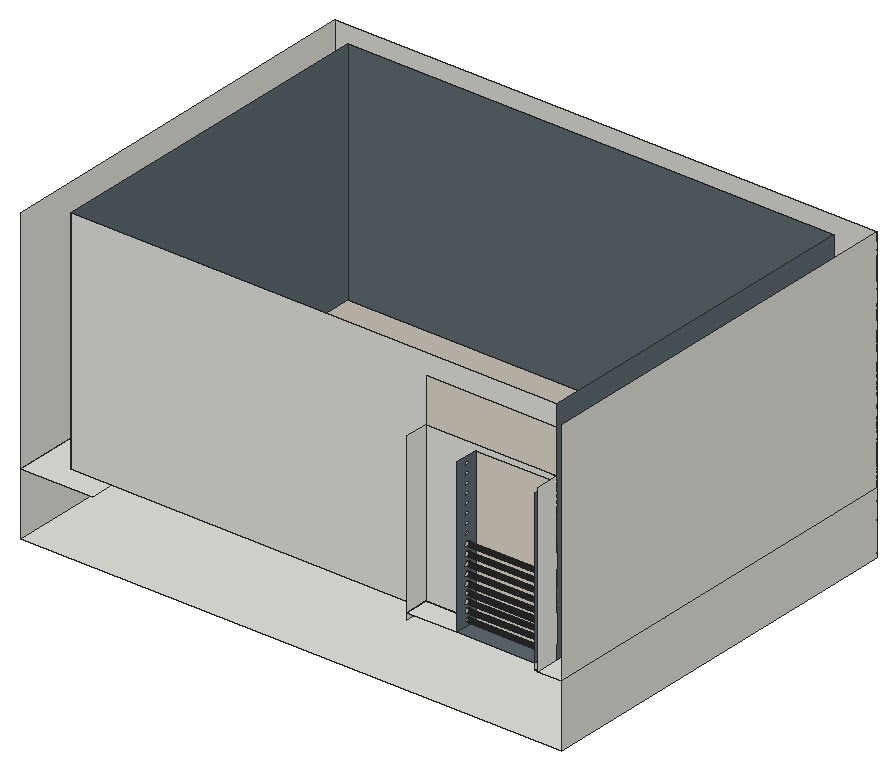
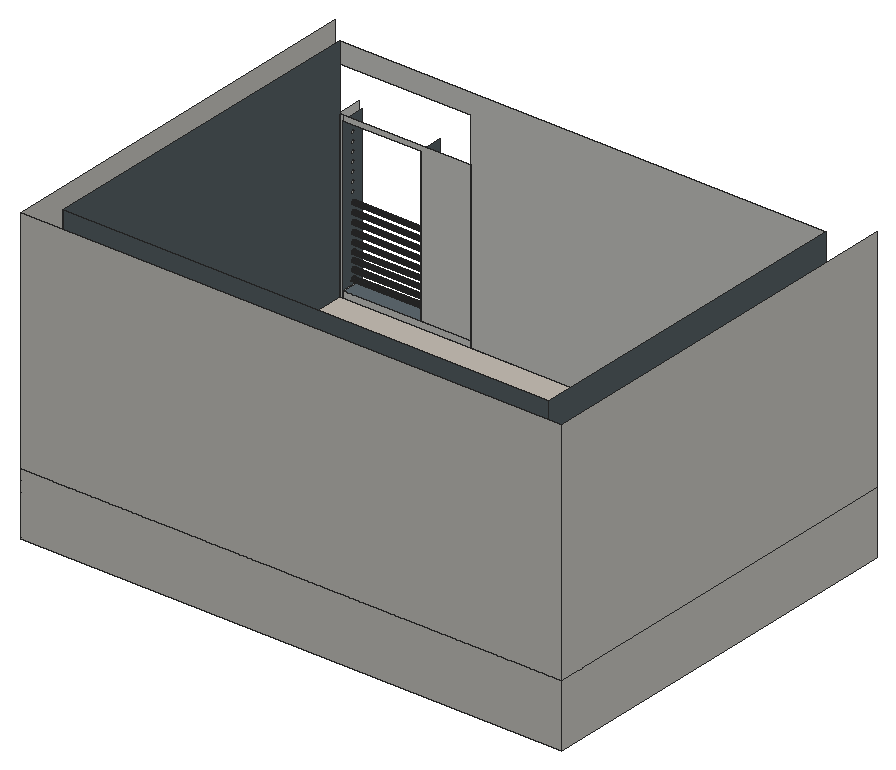
# SketchUp Ruby script. Lengths in inches.
U = 1.inch
M = Sketchup.active_model
def pt(a) = Geom::Point3d.new(a.map { |v| v * U })
def face(e, loops, mat)
  f = e.add_face(loops[0].map { |a| pt(a) })
  loops[1..].each { |l| e.add_face(l.map { |a| pt(a) }).erase! }
  f.material = f.back_material = mat if mat
  f
end
# faces: each face lists its corners as indices into pts; further lists are holes
def faces(e, pts, list, mat = nil) = list.each { |f| face(e, (f[0].is_a?(Array) ? f : [f]).map { |l| l.map { |i| pts[i] } }, mat) }
# xy, xz, yz: faces in a plane at the given z, y or x. An outline is a flat list of corners, or four numbers for a rectangle; further outlines are holes
def ring(l) = l.size == 4 ? [[l[0], l[1]], [l[2], l[1]], [l[2], l[3]], [l[0], l[3]]] : l.each_slice(2).to_a
def flat(e, list, mat, &to3) = list.each { |f| face(e, (f[0].is_a?(Array) ? f : [f]).map { |l| ring(l).map { |u, v| to3.(u, v) } }, mat) }
def xy(e, z, list, mat = nil) = flat(e, list, mat) { |x, y| [x, y, z] }
def xz(e, y, list, mat = nil) = flat(e, list, mat) { |x, z| [x, y, z] }
def yz(e, x, list, mat = nil) = flat(e, list, mat) { |y, z| [x, y, z] }
def lines(e, pts, list) = list.each { |a, b| e.add_line(pt(pts[a]), pt(pts[b])) }
# prism: a flat outline (further loops are holes) pulled along v
def prism(e, loops, v, mat = nil)
  f = face(e, loops, mat); d = Geom::Vector3d.new(v.map { |x| x * U })
  f.pushpull(f.normal.samedirection?(d) ? d.length : -d.length)
end
def box(e, o, s, mat = nil) = prism(e, [[o, [o[0] + s[0], o[1], o[2]], [o[0] + s[0], o[1] + s[1], o[2]], [o[0], o[1] + s[1], o[2]]]], [0, 0, s[2]], mat)
def at(x, y, z, deg = 0) = Geom::Transformation.translation(pt([x, y, z])) * Geom::Transformation.rotation(ORIGIN, Z_AXIS, deg.degrees)
def axes(o, x, y, z) = Geom::Transformation.new([*x, 0, *y, 0, *z, 0, *pt(o).to_a, 1])
def part(name) = M.definitions.add(name)
# library, detail: a bought-in or finely detailed component or shape, given as its bounding box
def library(name, o, s) = part(name).tap { |d| box(d.entities, o, s) }
def detail(e, o, s) = box(e.add_group.entities, o, s)
def put(e, d, t, mat = nil) = e.add_instance(d, t).tap { |i| i.material = mat if mat }
def group(e, t, mat = nil) = e.add_group.tap { |g| g.transformation = t; g.material = mat if mat }.entities
root = M.entities
M.materials.add("[Field Rectangle Tile]").color = [196, 189, 179]
M.materials.add("[Formica Laminate Dark]").color = [50, 53, 60]
M.materials.add("[Formica Speckled Grey]").color = [94, 105, 111]
M.materials.add("[Terrazzo Tile Light]").color = [219, 217, 210]
xy(root,0,[[57.16,175.06,340.49,380.73]])
xy(root,32.8125,[[57.16,175.06,57.16,380.73,340.49,380.73,340.49,175.06,328.05,175.06,328.05,368.29,73.72,368.29,73.72,187.5,94.84,187.5,94.84,175.06],[326.14,175.06,328.05,187.5]])
xy(root,32.8125,[[73.72,187.5,328.05,368.29]],"[Field Rectangle Tile]")
xy(root,36.375,[[259.37,175.06,285.76,187.5]])
xy(root,36.375,[[285.76,175.06,326.14,187.5]],"[Formica Speckled Grey]")
xz(root,187.5,[[73.72,32.8125,73.72,152.8125,328.05,152.8125,328.05,142.25,259.37,142.25,259.37,32.8125],[259.37,32.8125,326.14,36.375],[326.14,32.8125,328.05,119],[259.37,36.375,259.37,119,326.14,119,326.14,116.03,285.76,116.03,285.76,36.375]])
xz(root,368.29,[[73.72,32.8125,328.05,152.8125]],"[Formica Speckled Grey]")
xz(root,380.73,[[57.16,0,340.49,32.8125],[57.16,32.8125,340.49,152.8125]],"[Terrazzo Tile Light]")
yz(root,57.16,[[175.06,0,380.73,32.8125],[175.06,32.8125,380.73,152.8125]],"[Terrazzo Tile Light]")
yz(root,73.72,[[187.5,32.8125,368.29,152.8125]],"[Formica Speckled Grey]")
yz(root,259.37,[[175.06,32.8125,187.5,36.375],[175.06,36.375,187.5,119]])
yz(root,285.76,[[181.41,38.33,181.12,38.37,180.85,38.48,180.62,38.66,180.4375,38.9,180.33,39.17,180.29,39.46,180.33,39.75,180.4375,40.02,180.62,40.25,180.85,40.43,181.12,40.55,181.41,40.58,181.7,40.55,181.98,40.43,182.21,40.25,182.39,40.02,182.5,39.75,182.54,39.46,182.5,39.17,182.39,38.9,182.21,38.66,181.98,38.48,181.7,38.37],[181.28,42.8,180.99,42.84,180.72,42.95,180.49,43.125,180.31,43.36,180.2,43.63,180.16,43.92,180.2,44.21,180.31,44.48,180.49,44.72,180.72,44.9,180.99,45.01,181.28,45.05,181.57,45.01,181.84,44.9,182.08,44.72,182.26,44.48,182.37,44.21,182.41,43.92,182.37,43.63,182.26,43.36,182.08,43.125,181.84,42.95,181.57,42.84],[181.25,47.03,180.96,47.07,180.6875,47.18,180.45,47.36,180.28,47.59,180.16,47.86,180.125,48.15,180.16,48.44,180.28,48.72,180.45,48.95,180.6875,49.13,180.96,49.24,181.25,49.28,181.54,49.24,181.8125,49.13,182.05,48.95,182.22,48.72,182.34,48.44,182.375,48.15,182.34,47.86,182.22,47.59,182.05,47.36,181.8125,47.18,181.54,47.07],[181.25,51.09,180.96,51.13,180.6875,51.24,180.45,51.42,180.28,51.65,180.16,51.92,180.125,52.22,180.16,52.51,180.28,52.78,180.45,53.01,180.6875,53.19,180.96,53.3,181.25,53.34,181.54,53.3,181.8125,53.19,182.05,53.01,182.22,52.78,182.34,52.51,182.375,52.22,182.34,51.92,182.22,51.65,182.05,51.42,181.8125,51.24,181.54,51.13],[181.25,55.47,180.96,55.5,180.6875,55.62,180.45,55.8,180.28,56.03,180.16,56.3,180.125,56.59,180.16,56.88,180.28,57.15,180.45,57.39,180.6875,57.57,180.96,57.68,181.25,57.72,181.54,57.68,181.8125,57.57,182.05,57.39,182.22,57.15,182.34,56.88,182.375,56.59,182.34,56.3,182.22,56.03,182.05,55.8,181.8125,55.62,181.54,55.5],
  [181.25,60.15,180.96,60.19,180.6875,60.3,180.45,60.48,180.28,60.72,180.16,60.99,180.125,61.28,180.16,61.57,180.28,61.84,180.45,62.07,180.6875,62.25,180.96,62.37,181.25,62.4,181.54,62.37,181.8125,62.25,182.05,62.07,182.22,61.84,182.34,61.57,182.375,61.28,182.34,60.99,182.22,60.72,182.05,60.48,181.8125,60.3,181.54,60.19],[181.25,64.84,180.96,64.88,180.6875,64.99,180.45,65.17,180.28,65.4,180.16,65.67,180.125,65.97,180.16,66.26,180.28,66.53,180.45,66.76,180.6875,66.94,180.96,67.05,181.25,67.09,181.54,67.05,181.8125,66.94,182.05,66.76,182.22,66.53,182.34,66.26,182.375,65.97,182.34,65.67,182.22,65.4,182.05,65.17,181.8125,64.99,181.54,64.88],[181.25,69.53,180.96,69.57,180.6875,69.68,180.45,69.86,180.28,70.09,180.16,70.36,180.125,70.65,180.16,70.94,180.28,71.22,180.45,71.45,180.6875,71.63,180.96,71.74,181.25,71.78,181.54,71.74,181.8125,71.63,182.05,71.45,182.22,71.22,182.34,70.94,182.375,70.65,182.34,70.36,182.22,70.09,182.05,69.86,181.8125,69.68,181.54,69.57],[181.25,74.22,180.96,74.25,180.6875,74.37,180.45,74.55,180.28,74.78,180.16,75.05,180.125,75.34,180.16,75.63,180.28,75.9,180.45,76.14,180.6875,76.32,180.96,76.43,181.25,76.47,181.54,76.43,181.8125,76.32,182.05,76.14,182.22,75.9,182.34,75.63,182.375,75.34,182.34,75.05,182.22,74.78,182.05,74.55,181.8125,74.37,181.54,74.25]])
yz(root,285.76,[[[175.06,36.375,187.5,116.03],[181.25,107.03,180.96,107.07,180.6875,107.18,180.45,107.36,180.28,107.59,180.16,107.86,180.125,108.15,180.16,108.44,180.28,108.72,180.45,108.95,180.6875,109.13,180.96,109.24,181.25,109.28,181.54,109.24,181.8125,109.13,182.05,108.95,182.22,108.72,182.34,108.44,182.375,108.15,182.34,107.86,182.22,107.59,182.05,107.36,181.8125,107.18,181.54,107.07],[181.25,102.34,180.96,102.38,180.6875,102.49,180.45,102.67,180.28,102.9,180.16,103.17,180.125,103.47,180.16,103.76,180.28,104.03,180.45,104.26,180.6875,104.44,180.96,104.55,181.25,104.59,181.54,104.55,181.8125,104.44,182.05,104.26,182.22,104.03,182.34,103.76,182.375,103.47,182.34,103.17,182.22,102.9,182.05,102.67,181.8125,102.49,181.54,102.38],[181.25,97.65,180.96,97.69,180.6875,97.8,180.45,97.98,180.28,98.22,180.16,98.49,180.125,98.78,180.16,99.07,180.28,99.34,180.45,99.57,180.6875,99.75,180.96,99.87,181.25,99.9,181.54,99.87,181.8125,99.75,182.05,99.57,182.22,99.34,182.34,99.07,182.375,98.78,182.34,98.49,182.22,98.22,182.05,97.98,181.8125,97.8,181.54,97.69],[181.25,92.97,180.96,93,180.6875,93.12,180.45,93.3,180.28,93.53,180.16,93.8,180.125,94.09,180.16,94.38,180.28,94.65,180.45,94.89,180.6875,95.07,180.96,95.18,181.25,95.22,181.54,95.18,181.8125,95.07,182.05,94.89,182.22,94.65,182.34,94.38,182.375,94.09,182.34,93.8,182.22,93.53,182.05,93.3,181.8125,93.12,181.54,93],[181.25,88.28,180.96,88.32,180.6875,88.43,180.45,88.61,180.28,88.84,180.16,89.11,180.125,89.4,180.16,89.69,180.28,89.97,180.45,90.2,180.6875,90.38,180.96,90.49,181.25,90.53,181.54,90.49,181.8125,90.38,182.05,90.2,182.22,89.97,182.34,89.69,182.375,89.4,182.34,89.11,182.22,88.84,182.05,88.61,181.8125,88.43,181.54,88.32],[181.25,83.59,180.96,83.63,180.6875,83.74,180.45,83.92,180.28,84.15,180.16,84.42,180.125,84.72,180.16,85.01,180.28,85.28,180.45,85.51,180.6875,85.69,180.96,85.8,181.25,85.84,181.54,85.8,181.8125,85.69,182.05,85.51,182.22,85.28,182.34,85.01,182.375,84.72,182.34,84.42,182.22,84.15,182.05,83.92,181.8125,83.74,181.54,83.63],[181.25,78.9,180.96,78.94,180.6875,79.05,180.45,79.23,180.28,79.47,180.16,79.74,180.125,80.03,180.16,80.32,180.28,80.59,180.45,80.82,180.6875,81,180.96,81.12,181.25,81.15,181.54,81.12,181.8125,81,182.05,80.82,182.22,80.59,182.34,80.32,182.375,80.03,182.34,79.74,182.22,79.47,182.05,79.23,181.8125,79.05,181.54,78.94],[181.25,74.22,180.96,74.25,180.6875,74.37,180.45,74.55,180.28,74.78,180.16,75.05,180.125,75.34,180.16,75.63,180.28,75.9,180.45,76.14,180.6875,76.32,180.96,76.43,181.25,76.47,181.54,76.43,181.8125,76.32,182.05,76.14,182.22,75.9,182.34,75.63,182.375,75.34,182.34,75.05,182.22,74.78,182.05,74.55,181.8125,74.37,181.54,74.25],[181.25,69.53,180.96,69.57,180.6875,69.68,180.45,69.86,180.28,70.09,180.16,70.36,180.125,70.65,180.16,70.94,180.28,71.22,180.45,71.45,180.6875,71.63,180.96,71.74,181.25,71.78,181.54,71.74,181.8125,71.63,182.05,71.45,182.22,71.22,182.34,70.94,182.375,70.65,182.34,70.36,182.22,70.09,182.05,69.86,181.8125,69.68,181.54,69.57],[181.25,64.84,180.96,64.88,180.6875,64.99,180.45,65.17,180.28,65.4,180.16,65.67,180.125,65.97,180.16,66.26,180.28,66.53,180.45,66.76,180.6875,66.94,180.96,67.05,181.25,67.09,181.54,67.05,181.8125,66.94,182.05,66.76,182.22,66.53,182.34,66.26,182.375,65.97,182.34,65.67,182.22,65.4,182.05,65.17,181.8125,64.99,181.54,64.88],[181.25,60.15,180.96,60.19,180.6875,60.3,180.45,60.48,180.28,60.72,180.16,60.99,180.125,61.28,180.16,61.57,180.28,61.84,180.45,62.07,180.6875,62.25,180.96,62.37,181.25,62.4,181.54,62.37,181.8125,62.25,182.05,62.07,182.22,61.84,182.34,61.57,182.375,61.28,182.34,60.99,182.22,60.72,182.05,60.48,181.8125,60.3,181.54,60.19],[181.25,55.47,180.96,55.5,180.6875,55.62,180.45,55.8,180.28,56.03,180.16,56.3,180.125,56.59,180.16,56.88,180.28,57.15,180.45,57.39,180.6875,57.57,180.96,57.68,181.25,57.72,181.54,57.68,181.8125,57.57,182.05,57.39,182.22,57.15,182.34,56.88,182.375,56.59,182.34,56.3,182.22,56.03,182.05,55.8,181.8125,55.62,181.54,55.5],[181.41,38.33,181.12,38.37,180.85,38.48,180.62,38.66,180.4375,38.9,180.33,39.17,180.29,39.46,180.33,39.75,180.4375,40.02,180.62,40.25,180.85,40.43,181.12,40.55,181.41,40.58,181.7,40.55,181.98,40.43,182.21,40.25,182.39,40.02,182.5,39.75,182.54,39.46,182.5,39.17,182.39,38.9,182.21,38.66,181.98,38.48,181.7,38.37],[181.25,51.09,180.96,51.13,180.6875,51.24,180.45,51.42,180.28,51.65,180.16,51.92,180.125,52.22,180.16,52.51,180.28,52.78,180.45,53.01,180.6875,53.19,180.96,53.3,181.25,53.34,181.54,53.3,181.8125,53.19,182.05,53.01,182.22,52.78,182.34,52.51,182.375,52.22,182.34,51.92,182.22,51.65,182.05,51.42,181.8125,51.24,181.54,51.13],[181.28,42.8,180.99,42.84,180.72,42.95,180.49,43.125,180.31,43.36,180.2,43.63,180.16,43.92,180.2,44.21,180.31,44.48,180.49,44.72,180.72,44.9,180.99,45.01,181.28,45.05,181.57,45.01,181.84,44.9,182.08,44.72,182.26,44.48,182.37,44.21,182.41,43.92,182.37,43.63,182.26,43.36,182.08,43.125,181.84,42.95,181.57,42.84],[181.25,47.03,180.96,47.07,180.6875,47.18,180.45,47.36,180.28,47.59,180.16,47.86,180.125,48.15,180.16,48.44,180.28,48.72,180.45,48.95,180.6875,49.13,180.96,49.24,181.25,49.28,181.54,49.24,181.8125,49.13,182.05,48.95,182.22,48.72,182.34,48.44,182.375,48.15,182.34,47.86,182.22,47.59,182.05,47.36,181.8125,47.18,181.54,47.07],[181.25,111.72,180.96,111.75,180.6875,111.87,180.45,112.05,180.28,112.28,180.16,112.55,180.125,112.84,180.16,113.13,180.28,113.4,180.45,113.64,180.6875,113.82,180.96,113.93,181.25,113.97,181.54,113.93,181.8125,113.82,182.05,113.64,182.22,113.4,182.34,113.13,182.375,112.84,182.34,112.55,182.22,112.28,182.05,112.05,181.8125,111.87,181.54,111.75]]],"[Formica Speckled Grey]")
yz(root,326.14,[[175.06,32.8125,187.5,36.375]])
yz(root,326.14,[[[175.06,36.375,187.5,116.03],[181.25,111.72,181.54,111.75,181.8125,111.87,182.05,112.05,182.22,112.28,182.34,112.55,182.375,112.84,182.34,113.13,182.22,113.4,182.05,113.64,181.8125,113.82,181.54,113.93,181.25,113.97,180.96,113.93,180.6875,113.82,180.45,113.64,180.28,113.4,180.16,113.13,180.125,112.84,180.16,112.55,180.28,112.28,180.45,112.05,180.6875,111.87,180.96,111.75],[181.25,107.03,181.54,107.07,181.8125,107.18,182.05,107.36,182.22,107.59,182.34,107.86,182.375,108.15,182.34,108.44,182.22,108.72,182.05,108.95,181.8125,109.13,181.54,109.24,181.25,109.28,180.96,109.24,180.6875,109.13,180.45,108.95,180.28,108.72,180.16,108.44,180.125,108.15,180.16,107.86,180.28,107.59,180.45,107.36,180.6875,107.18,180.96,107.07],[181.25,102.34,181.54,102.38,181.8125,102.49,182.05,102.67,182.22,102.9,182.34,103.17,182.375,103.47,182.34,103.76,182.22,104.03,182.05,104.26,181.8125,104.44,181.54,104.55,181.25,104.59,180.96,104.55,180.6875,104.44,180.45,104.26,180.28,104.03,180.16,103.76,180.125,103.47,180.16,103.17,180.28,102.9,180.45,102.67,180.6875,102.49,180.96,102.38],[181.25,97.65,181.54,97.69,181.8125,97.8,182.05,97.98,182.22,98.22,182.34,98.49,182.375,98.78,182.34,99.07,182.22,99.34,182.05,99.57,181.8125,99.75,181.54,99.87,181.25,99.9,180.96,99.87,180.6875,99.75,180.45,99.57,180.28,99.34,180.16,99.07,180.125,98.78,180.16,98.49,180.28,98.22,180.45,97.98,180.6875,97.8,180.96,97.69],[181.25,92.97,181.54,93,181.8125,93.12,182.05,93.3,182.22,93.53,182.34,93.8,182.375,94.09,182.34,94.38,182.22,94.65,182.05,94.89,181.8125,95.07,181.54,95.18,181.25,95.22,180.96,95.18,180.6875,95.07,180.45,94.89,180.28,94.65,180.16,94.38,180.125,94.09,180.16,93.8,180.28,93.53,180.45,93.3,180.6875,93.12,180.96,93],[181.25,88.28,181.54,88.32,181.8125,88.43,182.05,88.61,182.22,88.84,182.34,89.11,182.375,89.4,182.34,89.69,182.22,89.97,182.05,90.2,181.8125,90.38,181.54,90.49,181.25,90.53,180.96,90.49,180.6875,90.38,180.45,90.2,180.28,89.97,180.16,89.69,180.125,89.4,180.16,89.11,180.28,88.84,180.45,88.61,180.6875,88.43,180.96,88.32],[181.25,83.59,181.54,83.63,181.8125,83.74,182.05,83.92,182.22,84.15,182.34,84.42,182.375,84.72,182.34,85.01,182.22,85.28,182.05,85.51,181.8125,85.69,181.54,85.8,181.25,85.84,180.96,85.8,180.6875,85.69,180.45,85.51,180.28,85.28,180.16,85.01,180.125,84.72,180.16,84.42,180.28,84.15,180.45,83.92,180.6875,83.74,180.96,83.63],[181.25,78.9,181.54,78.94,181.8125,79.05,182.05,79.23,182.22,79.47,182.34,79.74,182.375,80.03,182.34,80.32,182.22,80.59,182.05,80.82,181.8125,81,181.54,81.12,181.25,81.15,180.96,81.12,180.6875,81,180.45,80.82,180.28,80.59,180.16,80.32,180.125,80.03,180.16,79.74,180.28,79.47,180.45,79.23,180.6875,79.05,180.96,78.94],[181.25,74.22,181.54,74.25,181.8125,74.37,182.05,74.55,182.22,74.78,182.34,75.05,182.375,75.34,182.34,75.63,182.22,75.9,182.05,76.14,181.8125,76.32,181.54,76.43,181.25,76.47,180.96,76.43,180.6875,76.32,180.45,76.14,180.28,75.9,180.16,75.63,180.125,75.34,180.16,75.05,180.28,74.78,180.45,74.55,180.6875,74.37,180.96,74.25],[181.25,69.53,181.54,69.57,181.8125,69.68,182.05,69.86,182.22,70.09,182.34,70.36,182.375,70.65,182.34,70.94,182.22,71.22,182.05,71.45,181.8125,71.63,181.54,71.74,181.25,71.78,180.96,71.74,180.6875,71.63,180.45,71.45,180.28,71.22,180.16,70.94,180.125,70.65,180.16,70.36,180.28,70.09,180.45,69.86,180.6875,69.68,180.96,69.57],[181.25,64.84,181.54,64.88,181.8125,64.99,182.05,65.17,182.22,65.4,182.34,65.67,182.375,65.97,182.34,66.26,182.22,66.53,182.05,66.76,181.8125,66.94,181.54,67.05,181.25,67.09,180.96,67.05,180.6875,66.94,180.45,66.76,180.28,66.53,180.16,66.26,180.125,65.97,180.16,65.67,180.28,65.4,180.45,65.17,180.6875,64.99,180.96,64.88],[181.25,60.15,181.54,60.19,181.8125,60.3,182.05,60.48,182.22,60.72,182.34,60.99,182.375,61.28,182.34,61.57,182.22,61.84,182.05,62.07,181.8125,62.25,181.54,62.37,181.25,62.4,180.96,62.37,180.6875,62.25,180.45,62.07,180.28,61.84,180.16,61.57,180.125,61.28,180.16,60.99,180.28,60.72,180.45,60.48,180.6875,60.3,180.96,60.19],[181.25,55.47,181.54,55.5,181.8125,55.62,182.05,55.8,182.22,56.03,182.34,56.3,182.375,56.59,182.34,56.88,182.22,57.15,182.05,57.39,181.8125,57.57,181.54,57.68,181.25,57.72,180.96,57.68,180.6875,57.57,180.45,57.39,180.28,57.15,180.16,56.88,180.125,56.59,180.16,56.3,180.28,56.03,180.45,55.8,180.6875,55.62,180.96,55.5],[181.25,51.09,181.54,51.13,181.8125,51.24,182.05,51.42,182.22,51.65,182.34,51.92,182.375,52.22,182.34,52.51,182.22,52.78,182.05,53.01,181.8125,53.19,181.54,53.3,181.25,53.34,180.96,53.3,180.6875,53.19,180.45,53.01,180.28,52.78,180.16,52.51,180.125,52.22,180.16,51.92,180.28,51.65,180.45,51.42,180.6875,51.24,180.96,51.13],[181.25,47.03,181.54,47.07,181.8125,47.18,182.05,47.36,182.22,47.59,182.34,47.86,182.375,48.15,182.34,48.44,182.22,48.72,182.05,48.95,181.8125,49.13,181.54,49.24,181.25,49.28,180.96,49.24,180.6875,49.13,180.45,48.95,180.28,48.72,180.16,48.44,180.125,48.15,180.16,47.86,180.28,47.59,180.45,47.36,180.6875,47.18,180.96,47.07],[181.28,42.8,181.57,42.84,181.84,42.95,182.08,43.125,182.26,43.36,182.37,43.63,182.41,43.92,182.37,44.21,182.26,44.48,182.08,44.72,181.84,44.9,181.57,45.01,181.28,45.05,180.99,45.01,180.72,44.9,180.49,44.72,180.31,44.48,180.2,44.21,180.16,43.92,180.2,43.63,180.31,43.36,180.49,43.125,180.72,42.95,180.99,42.84],[181.41,38.33,181.7,38.37,181.98,38.48,182.21,38.66,182.39,38.9,182.5,39.17,182.54,39.46,182.5,39.75,182.39,40.02,182.21,40.25,181.98,40.43,181.7,40.55,181.41,40.58,181.12,40.55,180.85,40.43,180.62,40.25,180.4375,40.02,180.33,39.75,180.29,39.46,180.33,39.17,180.4375,38.9,180.62,38.66,180.85,38.48,181.12,38.37]]],"[Formica Speckled Grey]")
yz(root,328.05,[[175.06,32.8125,187.5,119]])
yz(root,328.05,[[187.5,32.8125,368.29,152.8125]],"[Formica Speckled Grey]")
yz(root,340.49,[[175.06,0,380.73,32.8125],[175.06,32.8125,380.73,152.8125]],"[Terrazzo Tile Light]")
p = [[285.76,181.12,38.37],[285.76,181.41,38.33],[326.14,181.41,38.33],[326.14,181.12,38.37],[285.76,181.7,38.37],[326.14,181.7,38.37],
  [285.76,181.98,38.48],[326.14,181.98,38.48],[285.76,182.21,38.66],[326.14,182.21,38.66],[285.76,182.39,38.9],[326.14,182.39,38.9],
  [285.76,182.5,39.17],[326.14,182.5,39.17],[285.76,182.54,39.46],[326.14,182.54,39.46],[285.76,182.5,39.75],[326.14,182.5,39.75],
  [285.76,182.39,40.02],[326.14,182.39,40.02],[285.76,182.21,40.25],[326.14,182.21,40.25],[285.76,181.98,40.43],[326.14,181.98,40.43],
  [285.76,181.7,40.55],[326.14,181.7,40.55],[285.76,181.41,40.58],[285.76,181.12,40.55],[326.14,181.12,40.55],[326.14,181.41,40.58],
  [285.76,180.99,42.84],[285.76,181.28,42.8],[326.14,181.28,42.8],[326.14,180.99,42.84],[285.76,181.57,42.84],[326.14,181.57,42.84],
  [285.76,181.84,42.95],[326.14,181.84,42.95],[285.76,182.08,43.125],[326.14,182.08,43.125],[285.76,182.26,43.36],[326.14,182.26,43.36],
  [285.76,182.37,43.63],[326.14,182.37,43.63],[285.76,182.41,43.92],[326.14,182.41,43.92],[285.76,182.37,44.21],[326.14,182.37,44.21],
  [285.76,182.26,44.48],[326.14,182.26,44.48],[285.76,182.08,44.72],[326.14,182.08,44.72],[285.76,181.84,44.9],[326.14,181.84,44.9],
  [285.76,181.57,45.01],[326.14,181.57,45.01],[285.76,181.28,45.05],[285.76,180.99,45.01],[326.14,180.99,45.01],[326.14,181.28,45.05],
  [285.76,181.25,47.03],[285.76,181.54,47.07],[326.14,181.54,47.07],[326.14,181.25,47.03],[285.76,181.8125,47.18],[326.14,181.8125,47.18],
  [285.76,182.05,47.36],[326.14,182.05,47.36],[285.76,182.22,47.59],[326.14,182.22,47.59],[285.76,182.34,47.86],[326.14,182.34,47.86],
  [285.76,182.375,48.15],[326.14,182.375,48.15],[285.76,182.34,48.44],[326.14,182.34,48.44],[285.76,182.22,48.72],[326.14,182.22,48.72],
  [285.76,182.05,48.95],[326.14,182.05,48.95],[285.76,181.8125,49.13],[326.14,181.8125,49.13],[285.76,181.54,49.24],[326.14,181.54,49.24],
  [285.76,181.25,49.28],[326.14,181.25,49.28],[285.76,180.96,51.13],[285.76,181.25,51.09],[326.14,181.25,51.09],[326.14,180.96,51.13],
  [285.76,181.54,51.13],[326.14,181.54,51.13],[285.76,181.8125,51.24],[326.14,181.8125,51.24],[285.76,182.05,51.42],[326.14,182.05,51.42],
  [285.76,182.22,51.65],[326.14,182.22,51.65],[285.76,182.34,51.92],[326.14,182.34,51.92],[285.76,182.375,52.22],[326.14,182.375,52.22],
  [285.76,182.34,52.51],[326.14,182.34,52.51],[285.76,182.22,52.78],[326.14,182.22,52.78],[285.76,182.05,53.01],[326.14,182.05,53.01],
  [285.76,181.8125,53.19],[326.14,181.8125,53.19],[285.76,181.54,53.3],[326.14,181.54,53.3],[285.76,181.25,53.34],[285.76,180.96,53.3],
  [326.14,180.96,53.3],[326.14,181.25,53.34],[285.76,180.96,55.5],[285.76,181.25,55.47],[326.14,181.25,55.47],[326.14,180.96,55.5],
  [285.76,181.54,55.5],[326.14,181.54,55.5],[285.76,181.8125,55.62],[326.14,181.8125,55.62],[285.76,182.05,55.8],[326.14,182.05,55.8],
  [285.76,182.22,56.03],[326.14,182.22,56.03],[285.76,182.34,56.3],[326.14,182.34,56.3],[285.76,182.375,56.59],[326.14,182.375,56.59],
  [285.76,182.34,56.88],[326.14,182.34,56.88],[285.76,182.22,57.15],[326.14,182.22,57.15],[285.76,182.05,57.39],[326.14,182.05,57.39],
  [285.76,181.8125,57.57],[326.14,181.8125,57.57],[285.76,181.54,57.68],[326.14,181.54,57.68],[285.76,181.25,57.72],[285.76,180.96,57.68],
  [326.14,180.96,57.68],[326.14,181.25,57.72],[285.76,180.96,60.19],[285.76,181.25,60.15],[326.14,181.25,60.15],[326.14,180.96,60.19],
  [285.76,181.54,60.19],[326.14,181.54,60.19],[285.76,181.8125,60.3],[326.14,181.8125,60.3],[285.76,182.05,60.48],[326.14,182.05,60.48],
  [285.76,182.22,60.72],[326.14,182.22,60.72],[285.76,182.34,60.99],[326.14,182.34,60.99],[285.76,182.375,61.28],[326.14,182.375,61.28],
  [285.76,182.34,61.57],[326.14,182.34,61.57],[285.76,182.22,61.84],[326.14,182.22,61.84],[285.76,182.05,62.07],[326.14,182.05,62.07],
  [285.76,181.8125,62.25],[326.14,181.8125,62.25],[285.76,181.54,62.37],[326.14,181.54,62.37],[285.76,181.25,62.4],[285.76,180.96,62.37],
  [326.14,180.96,62.37],[326.14,181.25,62.4],[285.76,180.96,64.88],[285.76,181.25,64.84],[326.14,181.25,64.84],[326.14,180.96,64.88],
  [285.76,181.54,64.88],[326.14,181.54,64.88],[285.76,181.8125,64.99],[326.14,181.8125,64.99],[285.76,182.05,65.17],[326.14,182.05,65.17],
  [285.76,182.22,65.4],[326.14,182.22,65.4],[285.76,182.34,65.67],[326.14,182.34,65.67],[285.76,182.375,65.97],[326.14,182.375,65.97],
  [285.76,182.34,66.26],[326.14,182.34,66.26],[285.76,182.22,66.53],[326.14,182.22,66.53],[285.76,182.05,66.76],[326.14,182.05,66.76],
  [285.76,181.8125,66.94],[326.14,181.8125,66.94],[285.76,181.54,67.05],[326.14,181.54,67.05],[285.76,181.25,67.09],[285.76,180.96,67.05],
  [326.14,180.96,67.05],[326.14,181.25,67.09],[285.76,180.96,69.57],[285.76,181.25,69.53],[326.14,181.25,69.53],[326.14,180.96,69.57],
  [285.76,181.54,69.57],[326.14,181.54,69.57],[285.76,181.8125,69.68],[326.14,181.8125,69.68],[285.76,182.05,69.86],[326.14,182.05,69.86],
  [285.76,182.22,70.09],[326.14,182.22,70.09],[285.76,182.34,70.36],[326.14,182.34,70.36],[285.76,182.375,70.65],[326.14,182.375,70.65],
  [285.76,182.34,70.94],[326.14,182.34,70.94],[285.76,182.22,71.22],[326.14,182.22,71.22],[285.76,182.05,71.45],[326.14,182.05,71.45],
  [285.76,181.8125,71.63],[326.14,181.8125,71.63],[285.76,181.54,71.74],[326.14,181.54,71.74],[285.76,181.25,71.78],[285.76,180.96,71.74],
  [326.14,180.96,71.74],[326.14,181.25,71.78],[285.76,180.96,74.25],[285.76,181.25,74.22],[326.14,181.25,74.22],[326.14,180.96,74.25],
  [285.76,181.54,74.25],[326.14,181.54,74.25],[285.76,181.8125,74.37],[326.14,181.8125,74.37],[285.76,182.05,74.55],[326.14,182.05,74.55],
  [285.76,182.22,74.78],[326.14,182.22,74.78],[285.76,182.34,75.05],[326.14,182.34,75.05],[285.76,182.375,75.34],[326.14,182.375,75.34],
  [285.76,182.34,75.63],[326.14,182.34,75.63],[285.76,182.22,75.9],[326.14,182.22,75.9],[285.76,182.05,76.14],[326.14,182.05,76.14],
  [285.76,181.8125,76.32],[326.14,181.8125,76.32],[285.76,181.54,76.43],[326.14,181.54,76.43],[285.76,181.25,76.47],[285.76,180.96,76.43],
  [326.14,180.96,76.43],[326.14,181.25,76.47]]
faces(root,p,[[0,1,2,3],[1,4,5,2],[4,6,7,5],[6,8,9,7],[8,10,11,9],[10,12,13,11],[12,14,15,13],[14,16,17,15],
  [16,18,19,17],[18,20,21,19],[20,22,23,21],[22,24,25,23],[26,27,28,29],[24,26,29,25],[30,31,32,33],[31,34,35,32],
  [34,36,37,35],[36,38,39,37],[38,40,41,39],[40,42,43,41],[42,44,45,43],[44,46,47,45],[46,48,49,47],[48,50,51,49],
  [50,52,53,51],[52,54,55,53],[56,57,58,59],[54,56,59,55],[60,61,62,63],[61,64,65,62],[64,66,67,65],[66,68,69,67],
  [68,70,71,69],[70,72,73,71],[72,74,75,73],[74,76,77,75],[76,78,79,77],[78,80,81,79],[80,82,83,81],[82,84,85,83],
  [86,87,88,89],[87,90,91,88],[90,92,93,91],[92,94,95,93],[94,96,97,95],[96,98,99,97],[98,100,101,99],[100,102,103,101],
  [102,104,105,103],[104,106,107,105],[106,108,109,107],[108,110,111,109],[112,113,114,115],[110,112,115,111],[116,117,118,119],[117,120,121,118],
  [120,122,123,121],[122,124,125,123],[124,126,127,125],[126,128,129,127],[128,130,131,129],[130,132,133,131],[132,134,135,133],[134,136,137,135],
  [136,138,139,137],[138,140,141,139],[142,143,144,145],[140,142,145,141],[146,147,148,149],[147,150,151,148],[150,152,153,151],[152,154,155,153],
  [154,156,157,155],[156,158,159,157],[158,160,161,159],[160,162,163,161],[162,164,165,163],[164,166,167,165],[166,168,169,167],[168,170,171,169],
  [172,173,174,175],[170,172,175,171],[176,177,178,179],[177,180,181,178],[180,182,183,181],[182,184,185,183],[184,186,187,185],[186,188,189,187],
  [188,190,191,189],[190,192,193,191],[192,194,195,193],[194,196,197,195],[196,198,199,197],[198,200,201,199],[202,203,204,205],[200,202,205,201],
  [206,207,208,209],[207,210,211,208],[210,212,213,211],[212,214,215,213],[214,216,217,215],[216,218,219,217],[218,220,221,219],[220,222,223,221],
  [222,224,225,223],[224,226,227,225],[226,228,229,227],[228,230,231,229],[232,233,234,235],[230,232,235,231],[236,237,238,239],[237,240,241,238],
  [240,242,243,241],[242,244,245,243],[244,246,247,245],[246,248,249,247],[248,250,251,249],[250,252,253,251],[252,254,255,253],[254,256,257,255],
  [256,258,259,257],[258,260,261,259],[262,263,264,265],[260,262,265,261]],"[Formica Laminate Dark]")
